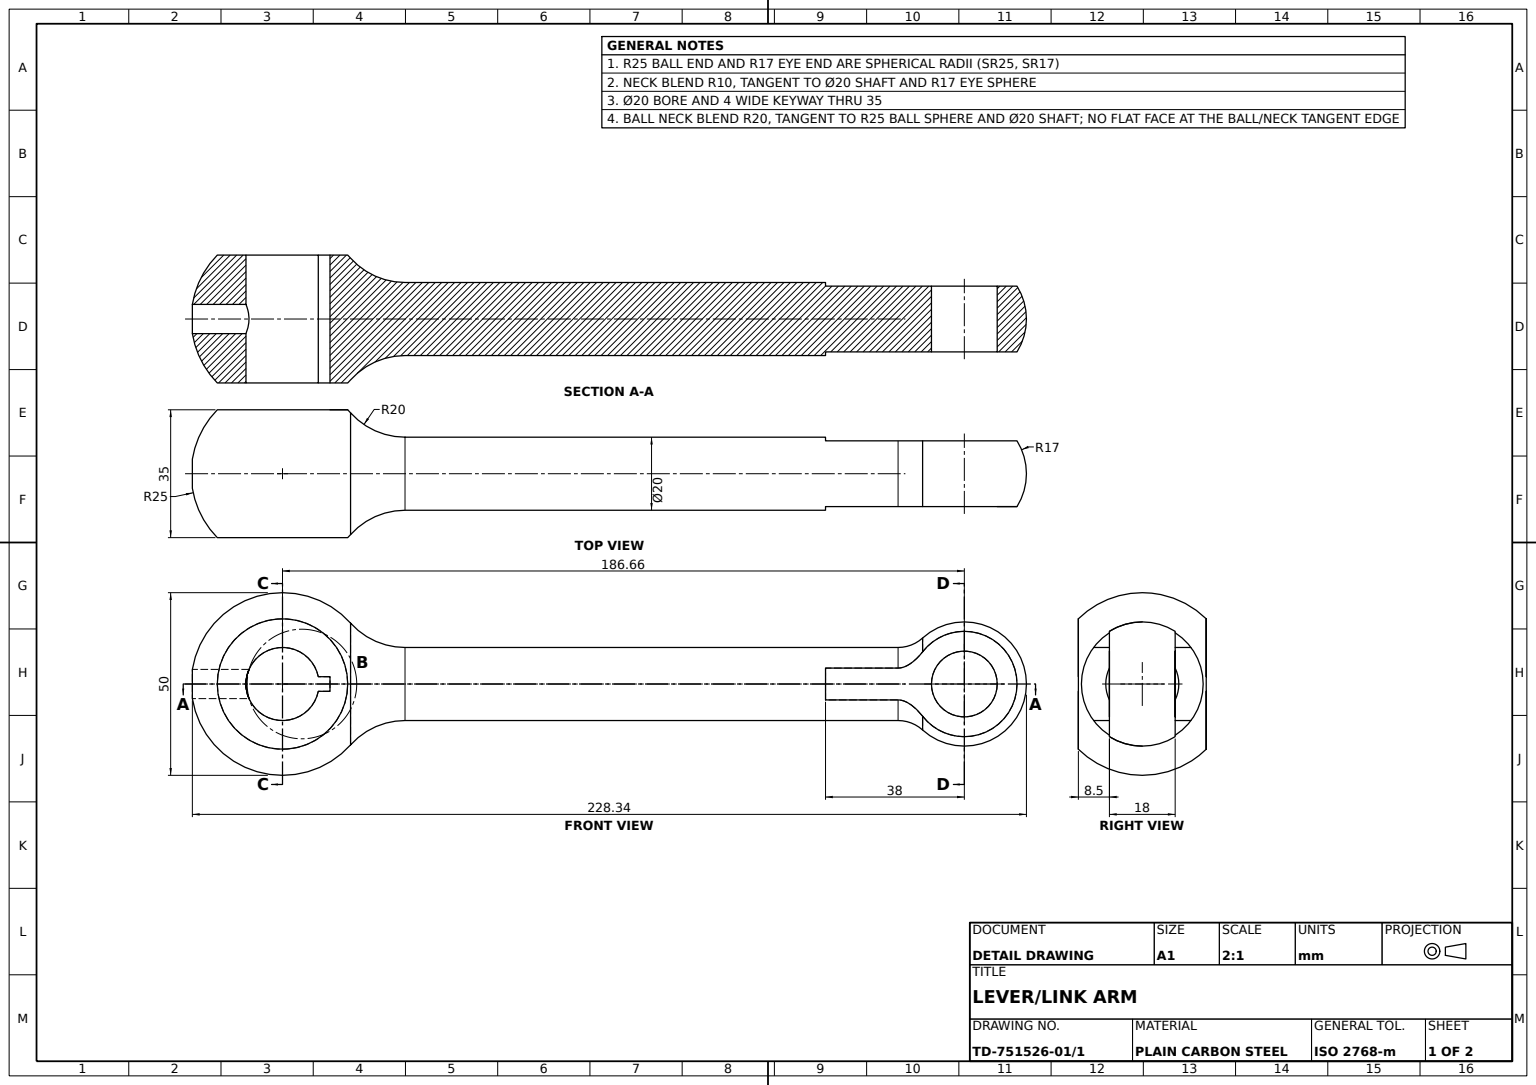
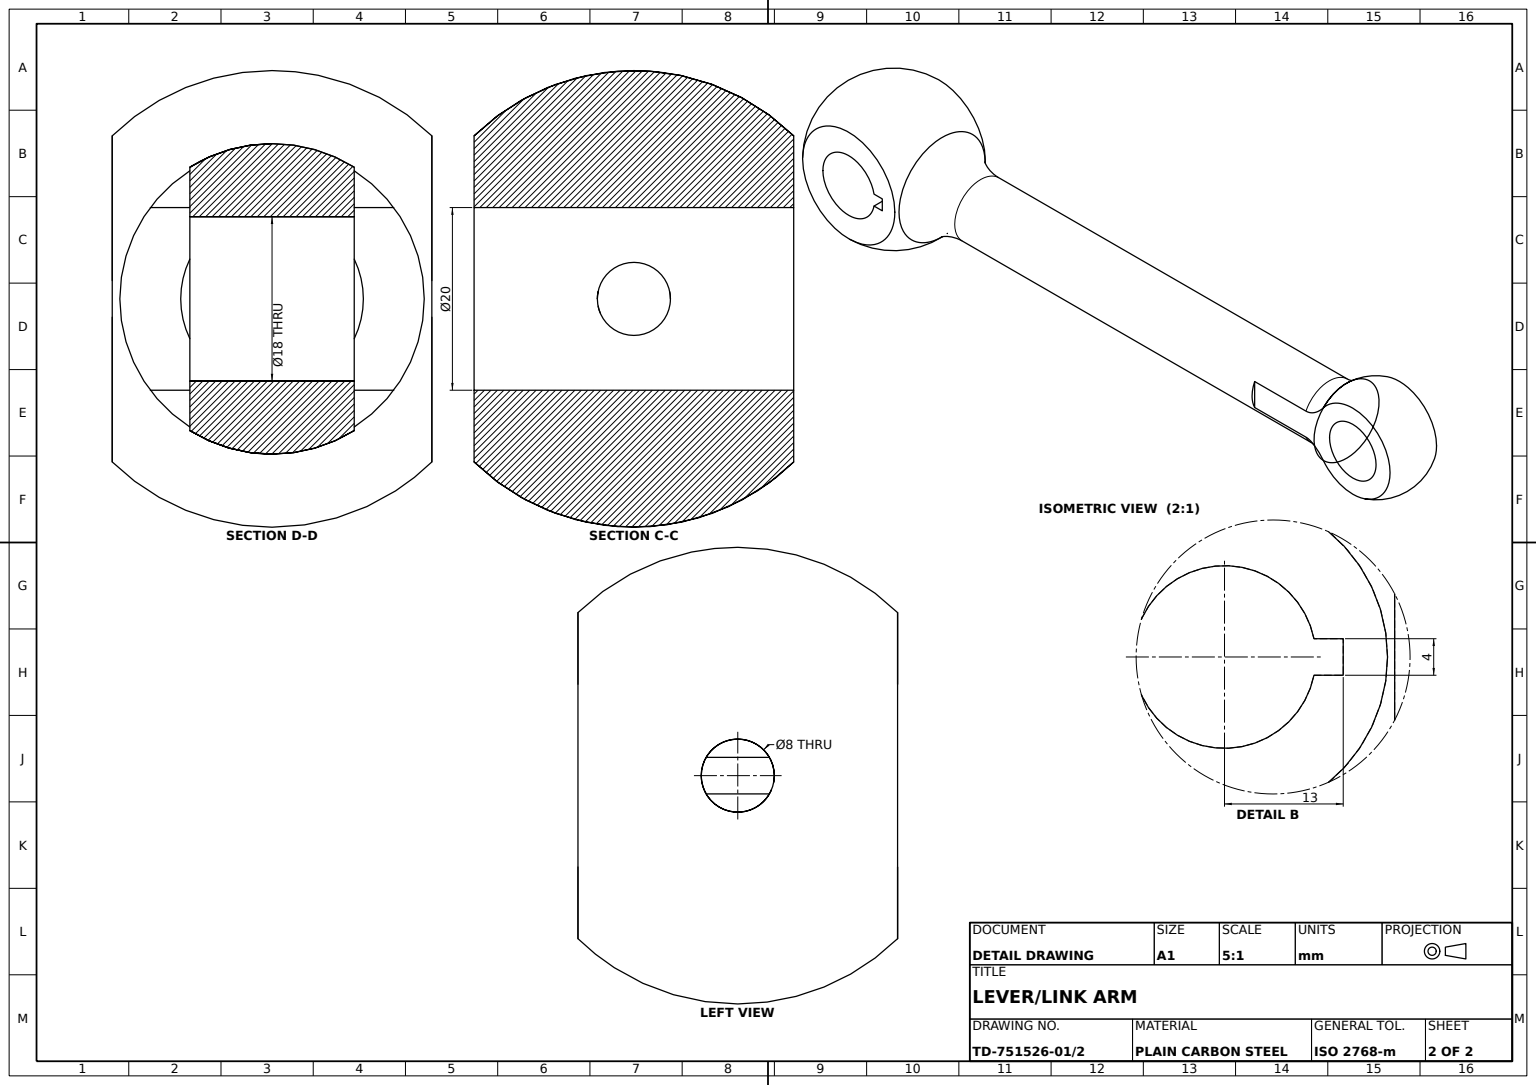
ISO-10303-21;
HEADER;
FILE_DESCRIPTION((''),'2;1');
FILE_NAME('','',(''),(''),'','','');
FILE_SCHEMA(('AUTOMOTIVE_DESIGN'));
ENDSEC;
DATA;
#1=APPLICATION_CONTEXT('');
#2=PRODUCT_CONTEXT('',#1,'mechanical');
#3=PRODUCT('','','',(#2));
#4=PRODUCT_DEFINITION_FORMATION('','',#3);
#5=PRODUCT_DEFINITION_CONTEXT('',#1,'design');
#6=PRODUCT_DEFINITION('','',#4,#5);
#7=PRODUCT_DEFINITION_SHAPE('','',#6);
#8=(LENGTH_UNIT()NAMED_UNIT(*)SI_UNIT(.MILLI.,.METRE.));
#9=(NAMED_UNIT(*)PLANE_ANGLE_UNIT()SI_UNIT($,.RADIAN.));
#10=(NAMED_UNIT(*)SI_UNIT($,.STERADIAN.)SOLID_ANGLE_UNIT());
#11=UNCERTAINTY_MEASURE_WITH_UNIT(LENGTH_MEASURE(1.E-05),#8,'distance_accuracy_value','');
#12=(GEOMETRIC_REPRESENTATION_CONTEXT(3)GLOBAL_UNCERTAINTY_ASSIGNED_CONTEXT((#11))GLOBAL_UNIT_ASSIGNED_CONTEXT((#8,#9,#10))REPRESENTATION_CONTEXT('',''));
#13=CARTESIAN_POINT('',(177.660606,0.,-9.));
#14=VERTEX_POINT('',#13);
#15=CARTESIAN_POINT('',(195.660606,0.,-9.));
#16=VERTEX_POINT('',#15);
#17=CARTESIAN_POINT('',(186.660606,0.,-9.));
#18=DIRECTION('',(0.,0.,-1.));
#19=DIRECTION('',(1.,0.,0.));
#20=AXIS2_PLACEMENT_3D('',#17,#18,#19);
#21=CIRCLE('',#20,9.);
#22=EDGE_CURVE('',#14,#16,#21,.T.);
#23=ORIENTED_EDGE('',*,*,#22,.T.);
#24=CARTESIAN_POINT('',(195.660606,0.,9.));
#25=VERTEX_POINT('',#24);
#26=CARTESIAN_POINT('',(195.660606,0.,-17.501));
#27=DIRECTION('',(0.,0.,1.));
#28=VECTOR('',#27,1000.);
#29=LINE('',#26,#28);
#30=EDGE_CURVE('',#16,#25,#29,.T.);
#31=ORIENTED_EDGE('',*,*,#30,.T.);
#32=CARTESIAN_POINT('',(177.660606,0.,9.));
#33=VERTEX_POINT('',#32);
#34=CARTESIAN_POINT('',(186.660606,0.,9.));
#35=AXIS2_PLACEMENT_3D('',#34,#27,#19);
#36=CIRCLE('',#35,9.);
#37=EDGE_CURVE('',#25,#33,#36,.T.);
#38=ORIENTED_EDGE('',*,*,#37,.T.);
#39=CARTESIAN_POINT('',(177.660606,0.,-17.501));
#40=LINE('',#39,#28);
#41=EDGE_CURVE('',#14,#33,#40,.T.);
#42=ORIENTED_EDGE('',*,*,#41,.F.);
#43=EDGE_LOOP('',(#23,#31,#38,#42));
#44=FACE_OUTER_BOUND('',#43,.T.);
#45=CARTESIAN_POINT('',(186.660606,0.,-17.501));
#46=AXIS2_PLACEMENT_3D('',#45,#27,#19);
#47=CYLINDRICAL_SURFACE('',#46,9.);
#48=ADVANCED_FACE('',(#44),#47,.F.);
#49=CARTESIAN_POINT('',(33.54102,0.,-10.));
#50=VERTEX_POINT('',#49);
#51=CARTESIAN_POINT('',(18.6339,0.,-16.666667));
#52=VERTEX_POINT('',#51);
#53=CARTESIAN_POINT('',(33.54102,0.,-30.));
#54=DIRECTION('',(0.,-1.,0.));
#55=AXIS2_PLACEMENT_3D('',#53,#54,#18);
#56=CIRCLE('',#55,20.);
#57=EDGE_CURVE('',#50,#52,#56,.T.);
#58=ORIENTED_EDGE('',*,*,#57,.T.);
#59=CARTESIAN_POINT('',(18.6339,0.,16.666667));
#60=VERTEX_POINT('',#59);
#61=CARTESIAN_POINT('',(18.6339,0.,0.));
#62=AXIS2_PLACEMENT_3D('',#61,#19,#18);
#63=CIRCLE('',#62,16.666667);
#64=EDGE_CURVE('',#52,#60,#63,.T.);
#65=ORIENTED_EDGE('',*,*,#64,.T.);
#66=CARTESIAN_POINT('',(33.54102,0.,10.));
#67=VERTEX_POINT('',#66);
#68=CARTESIAN_POINT('',(33.54102,0.,30.));
#69=DIRECTION('',(0.,1.,0.));
#70=AXIS2_PLACEMENT_3D('',#68,#69,#27);
#71=CIRCLE('',#70,20.);
#72=EDGE_CURVE('',#67,#60,#71,.T.);
#73=ORIENTED_EDGE('',*,*,#72,.F.);
#74=CARTESIAN_POINT('',(33.54102,0.,0.));
#75=AXIS2_PLACEMENT_3D('',#74,#19,#18);
#76=CIRCLE('',#75,10.);
#77=EDGE_CURVE('',#50,#67,#76,.T.);
#78=ORIENTED_EDGE('',*,*,#77,.F.);
#79=EDGE_LOOP('',(#58,#65,#73,#78));
#80=FACE_OUTER_BOUND('',#79,.T.);
#81=TOROIDAL_SURFACE('',#75,30.,20.);
#82=ADVANCED_FACE('',(#80),#81,.F.);
#83=ORIENTED_EDGE('',*,*,#30,.F.);
#84=EDGE_CURVE('',#16,#14,#21,.T.);
#85=ORIENTED_EDGE('',*,*,#84,.T.);
#86=ORIENTED_EDGE('',*,*,#41,.T.);
#87=EDGE_CURVE('',#33,#25,#36,.T.);
#88=ORIENTED_EDGE('',*,*,#87,.T.);
#89=EDGE_LOOP('',(#83,#85,#86,#88));
#90=FACE_OUTER_BOUND('',#89,.T.);
#91=ADVANCED_FACE('',(#90),#47,.F.);
#92=CARTESIAN_POINT('',(13.,2.,17.5));
#93=VERTEX_POINT('',#92);
#94=CARTESIAN_POINT('',(13.,-2.,17.5));
#95=VERTEX_POINT('',#94);
#96=VECTOR('',#54,1000.);
#97=LINE('',#92,#96);
#98=EDGE_CURVE('',#93,#95,#97,.T.);
#99=ORIENTED_EDGE('',*,*,#98,.F.);
#100=CARTESIAN_POINT('',(13.,2.,-17.5));
#101=VERTEX_POINT('',#100);
#102=CARTESIAN_POINT('',(13.,2.,17.501));
#103=VECTOR('',#18,1000.);
#104=LINE('',#102,#103);
#105=EDGE_CURVE('',#93,#101,#104,.T.);
#106=ORIENTED_EDGE('',*,*,#105,.T.);
#107=CARTESIAN_POINT('',(13.,-2.,-17.5));
#108=VERTEX_POINT('',#107);
#109=LINE('',#100,#96);
#110=EDGE_CURVE('',#101,#108,#109,.T.);
#111=ORIENTED_EDGE('',*,*,#110,.T.);
#112=CARTESIAN_POINT('',(13.,-2.,17.501));
#113=LINE('',#112,#103);
#114=EDGE_CURVE('',#95,#108,#113,.T.);
#115=ORIENTED_EDGE('',*,*,#114,.F.);
#116=EDGE_LOOP('',(#99,#106,#111,#115));
#117=FACE_OUTER_BOUND('',#116,.T.);
#118=AXIS2_PLACEMENT_3D('',#102,#19,#18);
#119=PLANE('',#118);
#120=ADVANCED_FACE('',(#117),#119,.F.);
#121=CARTESIAN_POINT('',(168.522248,4.358899,-9.));
#122=VERTEX_POINT('',#121);
#123=CARTESIAN_POINT('',(168.522248,4.358899,9.));
#124=VERTEX_POINT('',#123);
#125=CARTESIAN_POINT('',(168.522248,0.,0.));
#126=AXIS2_PLACEMENT_3D('',#125,#19,#18);
#127=CIRCLE('',#126,10.);
#128=EDGE_CURVE('',#122,#124,#127,.T.);
#129=ORIENTED_EDGE('',*,*,#128,.T.);
#130=CARTESIAN_POINT('',(175.240158,8.807576,9.));
#131=VERTEX_POINT('',#130);
#132=CARTESIAN_POINT('',(168.874076,4.358899,9.));
#133=CARTESIAN_POINT('',(169.21845,4.401685,9.));
#134=CARTESIAN_POINT('',(169.894624,4.559455,9.));
#135=CARTESIAN_POINT('',(170.22884,4.675527,9.));
#136=CARTESIAN_POINT('',(170.870066,4.956873,9.));
#137=CARTESIAN_POINT('',(171.175147,5.120207,9.));
#138=CARTESIAN_POINT('',(171.763901,5.478102,9.));
#139=CARTESIAN_POINT('',(172.047475,5.672809,9.));
#140=CARTESIAN_POINT('',(172.598036,6.086423,9.));
#141=CARTESIAN_POINT('',(172.864975,6.305399,9.));
#142=CARTESIAN_POINT('',(173.384701,6.763997,9.));
#143=CARTESIAN_POINT('',(173.638132,7.004413,9.));
#144=CARTESIAN_POINT('',(174.369091,7.744052,9.));
#145=CARTESIAN_POINT('',(174.820762,8.26376,9.));
#146=B_SPLINE_CURVE_WITH_KNOTS('',3,(#123,#132,#133,#134,#135,#136,#137,#138,#139,#140,#141,#142,#143,#144,#145,#130),.UNSPECIFIED.,.F.,.F.,(4,2,2,2,2,2,2,4),(0.066540398,0.067572352,0.068604305,0.069636258,0.070668212,0.071700165,0.072732118,0.074796025),.UNSPECIFIED.);
#147=EDGE_CURVE('',#124,#131,#146,.T.);
#148=ORIENTED_EDGE('',*,*,#147,.T.);
#149=CARTESIAN_POINT('',(175.240158,8.807576,-9.));
#150=VERTEX_POINT('',#149);
#151=CARTESIAN_POINT('',(175.240158,0.,0.));
#152=AXIS2_PLACEMENT_3D('',#151,#19,#18);
#153=CIRCLE('',#152,12.592593);
#154=EDGE_CURVE('',#150,#131,#153,.T.);
#155=ORIENTED_EDGE('',*,*,#154,.F.);
#156=CARTESIAN_POINT('',(168.874076,4.358899,-9.));
#157=CARTESIAN_POINT('',(169.21845,4.401685,-9.));
#158=CARTESIAN_POINT('',(169.894624,4.559455,-9.));
#159=CARTESIAN_POINT('',(170.22884,4.675527,-9.));
#160=CARTESIAN_POINT('',(170.870066,4.956873,-9.));
#161=CARTESIAN_POINT('',(171.175147,5.120207,-9.));
#162=CARTESIAN_POINT('',(171.763901,5.478102,-9.));
#163=CARTESIAN_POINT('',(172.047475,5.672809,-9.));
#164=CARTESIAN_POINT('',(172.598036,6.086423,-9.));
#165=CARTESIAN_POINT('',(172.864975,6.305399,-9.));
#166=CARTESIAN_POINT('',(173.384701,6.763997,-9.));
#167=CARTESIAN_POINT('',(173.638132,7.004413,-9.));
#168=CARTESIAN_POINT('',(174.369091,7.744052,-9.));
#169=CARTESIAN_POINT('',(174.820762,8.26376,-9.));
#170=B_SPLINE_CURVE_WITH_KNOTS('',3,(#121,#156,#157,#158,#159,#160,#161,#162,#163,#164,#165,#166,#167,#168,#169,#149),.UNSPECIFIED.,.F.,.F.,(4,2,2,2,2,2,2,4),(0.066540398,0.067572352,0.068604305,0.069636258,0.070668212,0.071700165,0.072732118,0.074796025),.UNSPECIFIED.);
#171=EDGE_CURVE('',#122,#150,#170,.T.);
#172=ORIENTED_EDGE('',*,*,#171,.F.);
#173=EDGE_LOOP('',(#129,#148,#155,#172));
#174=FACE_OUTER_BOUND('',#173,.T.);
#175=TOROIDAL_SURFACE('',#126,20.,10.);
#176=ADVANCED_FACE('',(#174),#175,.F.);
#177=CARTESIAN_POINT('',(-24.677925,0.,-4.));
#178=VERTEX_POINT('',#177);
#179=CARTESIAN_POINT('',(-17.853571,0.,-17.5));
#180=VERTEX_POINT('',#179);
#181=CARTESIAN_POINT('',(0.,0.,0.));
#182=AXIS2_PLACEMENT_3D('',#181,#54,#18);
#183=CIRCLE('',#182,25.);
#184=EDGE_CURVE('',#178,#180,#183,.T.);
#185=ORIENTED_EDGE('',*,*,#184,.F.);
#186=CARTESIAN_POINT('',(-24.677925,0.,4.));
#187=VERTEX_POINT('',#186);
#188=CARTESIAN_POINT('',(-24.677925,0.,0.));
#189=DIRECTION('',(-1.,0.,0.));
#190=AXIS2_PLACEMENT_3D('',#188,#189,#18);
#191=CIRCLE('',#190,4.);
#192=EDGE_CURVE('',#187,#178,#191,.T.);
#193=ORIENTED_EDGE('',*,*,#192,.F.);
#194=CARTESIAN_POINT('',(-17.853571,0.,17.5));
#195=VERTEX_POINT('',#194);
#196=AXIS2_PLACEMENT_3D('',#181,#69,#27);
#197=CIRCLE('',#196,25.);
#198=EDGE_CURVE('',#187,#195,#197,.T.);
#199=ORIENTED_EDGE('',*,*,#198,.T.);
#200=CARTESIAN_POINT('',(17.853571,0.,17.5));
#201=VERTEX_POINT('',#200);
#202=CARTESIAN_POINT('',(0.,0.,17.5));
#203=AXIS2_PLACEMENT_3D('',#202,#27,#19);
#204=CIRCLE('',#203,17.853571);
#205=EDGE_CURVE('',#201,#195,#204,.T.);
#206=ORIENTED_EDGE('',*,*,#205,.F.);
#207=EDGE_CURVE('',#201,#60,#197,.T.);
#208=ORIENTED_EDGE('',*,*,#207,.T.);
#209=ORIENTED_EDGE('',*,*,#64,.F.);
#210=CARTESIAN_POINT('',(17.853571,0.,-17.5));
#211=VERTEX_POINT('',#210);
#212=EDGE_CURVE('',#211,#52,#183,.T.);
#213=ORIENTED_EDGE('',*,*,#212,.F.);
#214=CARTESIAN_POINT('',(0.,0.,-17.5));
#215=AXIS2_PLACEMENT_3D('',#214,#27,#19);
#216=CIRCLE('',#215,17.853571);
#217=EDGE_CURVE('',#211,#180,#216,.T.);
#218=ORIENTED_EDGE('',*,*,#217,.T.);
#219=EDGE_LOOP('',(#185,#193,#199,#206,#208,#209,#213,#218));
#220=FACE_OUTER_BOUND('',#219,.T.);
#221=AXIS2_PLACEMENT_3D('',#181,#69,#18);
#222=SPHERICAL_SURFACE('',#221,25.);
#223=ADVANCED_FACE('',(#220),#222,.T.);
#224=ORIENTED_EDGE('',*,*,#22,.F.);
#225=ORIENTED_EDGE('',*,*,#84,.F.);
#226=EDGE_LOOP('',(#224,#225));
#227=FACE_BOUND('',#226,.T.);
#228=CARTESIAN_POINT('',(148.660606,4.358899,-9.));
#229=VERTEX_POINT('',#228);
#230=CARTESIAN_POINT('',(248.139692,4.358899,-9.));
#231=VECTOR('',#19,1000.);
#232=LINE('',#230,#231);
#233=EDGE_CURVE('',#229,#122,#232,.T.);
#234=ORIENTED_EDGE('',*,*,#233,.T.);
#235=ORIENTED_EDGE('',*,*,#171,.T.);
#236=CARTESIAN_POINT('',(201.082811,0.,-9.));
#237=VERTEX_POINT('',#236);
#238=CIRCLE('',#20,14.422205);
#239=EDGE_CURVE('',#150,#237,#238,.T.);
#240=ORIENTED_EDGE('',*,*,#239,.T.);
#241=CARTESIAN_POINT('',(175.240158,-8.807576,-9.));
#242=VERTEX_POINT('',#241);
#243=EDGE_CURVE('',#237,#242,#238,.T.);
#244=ORIENTED_EDGE('',*,*,#243,.T.);
#245=CARTESIAN_POINT('',(168.522248,-4.358899,-9.));
#246=VERTEX_POINT('',#245);
#247=CARTESIAN_POINT('',(174.81656,-8.258312,-9.));
#248=CARTESIAN_POINT('',(174.36214,-7.736405,-9.));
#249=CARTESIAN_POINT('',(173.38727,-6.751194,-9.));
#250=CARTESIAN_POINT('',(172.867869,-6.288445,-9.));
#251=CARTESIAN_POINT('',(172.038646,-5.66653,-9.));
#252=CARTESIAN_POINT('',(171.753259,-5.470946,-9.));
#253=CARTESIAN_POINT('',(171.158648,-5.110896,-9.));
#254=CARTESIAN_POINT('',(170.85143,-4.94783,-9.));
#255=CARTESIAN_POINT('',(170.218697,-4.671983,-9.));
#256=CARTESIAN_POINT('',(169.892126,-4.558498,-9.));
#257=CARTESIAN_POINT('',(169.210806,-4.400281,-9.));
#258=CARTESIAN_POINT('',(168.867809,-4.358899,-9.));
#259=B_SPLINE_CURVE_WITH_KNOTS('',3,(#241,#247,#248,#249,#250,#251,#252,#253,#254,#255,#256,#257,#258,#245),.UNSPECIFIED.,.F.,.F.,(4,2,2,2,2,2,4),(0.066419466,0.068492414,0.070565363,0.071601837,0.072638311,0.073674786,0.07471126),.UNSPECIFIED.);
#260=EDGE_CURVE('',#242,#246,#259,.T.);
#261=ORIENTED_EDGE('',*,*,#260,.T.);
#262=CARTESIAN_POINT('',(148.660606,-4.358899,-9.));
#263=VERTEX_POINT('',#262);
#264=CARTESIAN_POINT('',(248.139692,-4.358899,-9.));
#265=VECTOR('',#189,1000.);
#266=LINE('',#264,#265);
#267=EDGE_CURVE('',#246,#263,#266,.T.);
#268=ORIENTED_EDGE('',*,*,#267,.T.);
#269=CARTESIAN_POINT('',(148.660606,5.,-9.));
#270=LINE('',#269,#96);
#271=EDGE_CURVE('',#229,#263,#270,.T.);
#272=ORIENTED_EDGE('',*,*,#271,.F.);
#273=EDGE_LOOP('',(#234,#235,#240,#244,#261,#268,#272));
#274=FACE_OUTER_BOUND('',#273,.T.);
#275=AXIS2_PLACEMENT_3D('',#17,#27,#19);
#276=PLANE('',#275);
#277=ADVANCED_FACE('',(#227,#274),#276,.F.);
#278=CARTESIAN_POINT('',(9.797959,-2.,17.5));
#279=VERTEX_POINT('',#278);
#280=LINE('',#94,#265);
#281=EDGE_CURVE('',#95,#279,#280,.T.);
#282=ORIENTED_EDGE('',*,*,#281,.F.);
#283=ORIENTED_EDGE('',*,*,#114,.T.);
#284=CARTESIAN_POINT('',(9.797959,-2.,-17.5));
#285=VERTEX_POINT('',#284);
#286=LINE('',#107,#265);
#287=EDGE_CURVE('',#108,#285,#286,.T.);
#288=ORIENTED_EDGE('',*,*,#287,.T.);
#289=CARTESIAN_POINT('',(9.797959,-2.,17.501));
#290=LINE('',#289,#103);
#291=EDGE_CURVE('',#279,#285,#290,.T.);
#292=ORIENTED_EDGE('',*,*,#291,.F.);
#293=EDGE_LOOP('',(#282,#283,#288,#292));
#294=FACE_OUTER_BOUND('',#293,.T.);
#295=AXIS2_PLACEMENT_3D('',#112,#54,#18);
#296=PLANE('',#295);
#297=ADVANCED_FACE('',(#294),#296,.F.);
#298=CARTESIAN_POINT('',(168.522248,-4.358899,9.));
#299=VERTEX_POINT('',#298);
#300=CARTESIAN_POINT('',(148.660606,-4.358899,9.));
#301=VERTEX_POINT('',#300);
#302=CARTESIAN_POINT('',(248.139692,-4.358899,9.));
#303=LINE('',#302,#265);
#304=EDGE_CURVE('',#299,#301,#303,.T.);
#305=ORIENTED_EDGE('',*,*,#304,.F.);
#306=CARTESIAN_POINT('',(175.240158,-8.807576,9.));
#307=VERTEX_POINT('',#306);
#308=CARTESIAN_POINT('',(174.81656,-8.258312,9.));
#309=CARTESIAN_POINT('',(174.36214,-7.736405,9.));
#310=CARTESIAN_POINT('',(173.38727,-6.751194,9.));
#311=CARTESIAN_POINT('',(172.867869,-6.288445,9.));
#312=CARTESIAN_POINT('',(172.038646,-5.66653,9.));
#313=CARTESIAN_POINT('',(171.753259,-5.470946,9.));
#314=CARTESIAN_POINT('',(171.158648,-5.110896,9.));
#315=CARTESIAN_POINT('',(170.85143,-4.94783,9.));
#316=CARTESIAN_POINT('',(170.218697,-4.671983,9.));
#317=CARTESIAN_POINT('',(169.892126,-4.558498,9.));
#318=CARTESIAN_POINT('',(169.210806,-4.400281,9.));
#319=CARTESIAN_POINT('',(168.867809,-4.358899,9.));
#320=B_SPLINE_CURVE_WITH_KNOTS('',3,(#306,#308,#309,#310,#311,#312,#313,#314,#315,#316,#317,#318,#319,#298),.UNSPECIFIED.,.F.,.F.,(4,2,2,2,2,2,4),(0.066419466,0.068492414,0.070565363,0.071601837,0.072638311,0.073674786,0.07471126),.UNSPECIFIED.);
#321=EDGE_CURVE('',#307,#299,#320,.T.);
#322=ORIENTED_EDGE('',*,*,#321,.F.);
#323=CARTESIAN_POINT('',(201.082811,0.,9.));
#324=VERTEX_POINT('',#323);
#325=AXIS2_PLACEMENT_3D('',#34,#18,#19);
#326=CIRCLE('',#325,14.422205);
#327=EDGE_CURVE('',#324,#307,#326,.T.);
#328=ORIENTED_EDGE('',*,*,#327,.F.);
#329=EDGE_CURVE('',#131,#324,#326,.T.);
#330=ORIENTED_EDGE('',*,*,#329,.F.);
#331=ORIENTED_EDGE('',*,*,#147,.F.);
#332=CARTESIAN_POINT('',(148.660606,4.358899,9.));
#333=VERTEX_POINT('',#332);
#334=CARTESIAN_POINT('',(248.139692,4.358899,9.));
#335=LINE('',#334,#231);
#336=EDGE_CURVE('',#333,#124,#335,.T.);
#337=ORIENTED_EDGE('',*,*,#336,.F.);
#338=CARTESIAN_POINT('',(148.660606,5.,9.));
#339=LINE('',#338,#96);
#340=EDGE_CURVE('',#333,#301,#339,.T.);
#341=ORIENTED_EDGE('',*,*,#340,.T.);
#342=EDGE_LOOP('',(#305,#322,#328,#330,#331,#337,#341));
#343=FACE_OUTER_BOUND('',#342,.T.);
#344=ORIENTED_EDGE('',*,*,#87,.F.);
#345=ORIENTED_EDGE('',*,*,#37,.F.);
#346=EDGE_LOOP('',(#344,#345));
#347=FACE_BOUND('',#346,.T.);
#348=PLANE('',#35);
#349=ADVANCED_FACE('',(#343,#347),#348,.T.);
#350=ORIENTED_EDGE('',*,*,#271,.T.);
#351=CARTESIAN_POINT('',(148.660606,0.,-10.));
#352=VERTEX_POINT('',#351);
#353=CARTESIAN_POINT('',(148.660606,0.,0.));
#354=AXIS2_PLACEMENT_3D('',#353,#19,#27);
#355=CIRCLE('',#354,10.);
#356=EDGE_CURVE('',#263,#352,#355,.T.);
#357=ORIENTED_EDGE('',*,*,#356,.T.);
#358=EDGE_CURVE('',#352,#229,#355,.T.);
#359=ORIENTED_EDGE('',*,*,#358,.T.);
#360=EDGE_LOOP('',(#350,#357,#359));
#361=FACE_OUTER_BOUND('',#360,.T.);
#362=CARTESIAN_POINT('',(148.660606,5.,-17.501));
#363=AXIS2_PLACEMENT_3D('',#362,#189,#27);
#364=PLANE('',#363);
#365=ADVANCED_FACE('',(#361),#364,.F.);
#366=EDGE_CURVE('',#60,#52,#63,.T.);
#367=ORIENTED_EDGE('',*,*,#366,.T.);
#368=ORIENTED_EDGE('',*,*,#57,.F.);
#369=EDGE_CURVE('',#67,#50,#76,.T.);
#370=ORIENTED_EDGE('',*,*,#369,.F.);
#371=ORIENTED_EDGE('',*,*,#72,.T.);
#372=EDGE_LOOP('',(#367,#368,#370,#371));
#373=FACE_OUTER_BOUND('',#372,.T.);
#374=ADVANCED_FACE('',(#373),#81,.F.);
#375=EDGE_CURVE('',#299,#246,#127,.T.);
#376=ORIENTED_EDGE('',*,*,#375,.T.);
#377=ORIENTED_EDGE('',*,*,#260,.F.);
#378=EDGE_CURVE('',#307,#242,#153,.T.);
#379=ORIENTED_EDGE('',*,*,#378,.F.);
#380=ORIENTED_EDGE('',*,*,#321,.T.);
#381=EDGE_LOOP('',(#376,#377,#379,#380));
#382=FACE_OUTER_BOUND('',#381,.T.);
#383=ADVANCED_FACE('',(#382),#175,.F.);
#384=CARTESIAN_POINT('',(-10.,0.,4.));
#385=VERTEX_POINT('',#384);
#386=CARTESIAN_POINT('',(-10.,0.,-4.));
#387=VERTEX_POINT('',#386);
#388=CARTESIAN_POINT('',(-10.,-0.263112,4.));
#389=CARTESIAN_POINT('',(-9.989336,-0.52985,3.973555));
#390=CARTESIAN_POINT('',(-9.948313,-1.048164,3.869268));
#391=CARTESIAN_POINT('',(-9.918356,-1.298524,3.792435));
#392=CARTESIAN_POINT('',(-9.842917,-1.782398,3.590513));
#393=CARTESIAN_POINT('',(-9.797311,-2.015291,3.464932));
#394=CARTESIAN_POINT('',(-9.698876,-2.445507,3.175948));
#395=CARTESIAN_POINT('',(-9.645461,-2.646134,3.010987));
#396=CARTESIAN_POINT('',(-9.536652,-3.014832,2.641753));
#397=CARTESIAN_POINT('',(-9.482634,-3.178513,2.442105));
#398=CARTESIAN_POINT('',(-9.381221,-3.466408,2.012671));
#399=CARTESIAN_POINT('',(-9.333353,-3.591691,1.779932));
#400=CARTESIAN_POINT('',(-9.25342,-3.792879,1.2971));
#401=CARTESIAN_POINT('',(-9.221268,-3.86929,1.047714));
#402=CARTESIAN_POINT('',(-9.177005,-3.973131,0.532297));
#403=CARTESIAN_POINT('',(-9.165166,-3.999967,0.264113));
#404=CARTESIAN_POINT('',(-9.165137,-4.000033,-0.263104));
#405=CARTESIAN_POINT('',(-9.176515,-3.974265,-0.525135));
#406=CARTESIAN_POINT('',(-9.220997,-3.869938,-1.046004));
#407=CARTESIAN_POINT('',(-9.253578,-3.792487,-1.298117));
#408=CARTESIAN_POINT('',(-9.33333,-3.591742,-1.779734));
#409=CARTESIAN_POINT('',(-9.381197,-3.46651,-2.012662));
#410=CARTESIAN_POINT('',(-9.483143,-3.177034,-2.444167));
#411=CARTESIAN_POINT('',(-9.537174,-3.013117,-2.643571));
#412=CARTESIAN_POINT('',(-9.645399,-2.646291,-3.010729));
#413=CARTESIAN_POINT('',(-9.699402,-2.443392,-3.177539));
#414=CARTESIAN_POINT('',(-9.797619,-2.013759,-3.465789));
#415=CARTESIAN_POINT('',(-9.842453,-1.785184,-3.58926));
#416=CARTESIAN_POINT('',(-9.918457,-1.298068,-3.792715));
#417=CARTESIAN_POINT('',(-9.948453,-1.046303,-3.869623));
#418=CARTESIAN_POINT('',(-9.989151,-0.532292,-3.973084));
#419=CARTESIAN_POINT('',(-10.,-0.267133,-4.));
#420=B_SPLINE_CURVE_WITH_KNOTS('',3,(#384,#388,#389,#390,#391,#392,#393,#394,#395,#396,#397,#398,#399,#400,#401,#402,#403,#404,#405,#406,#407,#408,#409,#410,#411,#412,#413,#414,#415,#416,#417,#418,#419,#386),.UNSPECIFIED.,.F.,.F.,(4,2,2,2,2,2,2,2,2,2,2,2,2,2,2,2,4),(0.012639562,0.013429016,0.014218471,0.015007925,0.015797379,0.016586833,0.017376287,0.018165741,0.018955196,0.01974465,0.020534104,0.021323558,0.022113012,0.022902467,0.023691921,0.024481375,0.025270829),.UNSPECIFIED.);
#421=EDGE_CURVE('',#385,#387,#420,.T.);
#422=ORIENTED_EDGE('',*,*,#421,.F.);
#423=CARTESIAN_POINT('',(-10.,0.,17.5));
#424=VERTEX_POINT('',#423);
#425=CARTESIAN_POINT('',(-10.,0.,17.501));
#426=LINE('',#425,#103);
#427=EDGE_CURVE('',#424,#385,#426,.T.);
#428=ORIENTED_EDGE('',*,*,#427,.F.);
#429=AXIS2_PLACEMENT_3D('',#202,#18,#19);
#430=CIRCLE('',#429,10.);
#431=EDGE_CURVE('',#279,#424,#430,.T.);
#432=ORIENTED_EDGE('',*,*,#431,.F.);
#433=ORIENTED_EDGE('',*,*,#291,.T.);
#434=CARTESIAN_POINT('',(-10.,0.,-17.5));
#435=VERTEX_POINT('',#434);
#436=AXIS2_PLACEMENT_3D('',#214,#18,#189);
#437=CIRCLE('',#436,10.);
#438=EDGE_CURVE('',#285,#435,#437,.T.);
#439=ORIENTED_EDGE('',*,*,#438,.T.);
#440=EDGE_CURVE('',#387,#435,#426,.T.);
#441=ORIENTED_EDGE('',*,*,#440,.F.);
#442=EDGE_LOOP('',(#422,#428,#432,#433,#439,#441));
#443=FACE_OUTER_BOUND('',#442,.T.);
#444=CARTESIAN_POINT('',(0.,0.,17.501));
#445=AXIS2_PLACEMENT_3D('',#444,#18,#189);
#446=CYLINDRICAL_SURFACE('',#445,10.);
#447=ADVANCED_FACE('',(#443),#446,.F.);
#448=ORIENTED_EDGE('',*,*,#243,.F.);
#449=CARTESIAN_POINT('',(203.660606,0.,0.));
#450=VERTEX_POINT('',#449);
#451=CARTESIAN_POINT('',(186.660606,0.,0.));
#452=AXIS2_PLACEMENT_3D('',#451,#54,#18);
#453=CIRCLE('',#452,17.);
#454=EDGE_CURVE('',#237,#450,#453,.T.);
#455=ORIENTED_EDGE('',*,*,#454,.T.);
#456=AXIS2_PLACEMENT_3D('',#451,#69,#27);
#457=CIRCLE('',#456,17.);
#458=EDGE_CURVE('',#324,#450,#457,.T.);
#459=ORIENTED_EDGE('',*,*,#458,.F.);
#460=ORIENTED_EDGE('',*,*,#327,.T.);
#461=ORIENTED_EDGE('',*,*,#378,.T.);
#462=EDGE_LOOP('',(#448,#455,#459,#460,#461));
#463=FACE_OUTER_BOUND('',#462,.T.);
#464=AXIS2_PLACEMENT_3D('',#451,#54,#27);
#465=SPHERICAL_SURFACE('',#464,17.);
#466=ADVANCED_FACE('',(#463),#465,.T.);
#467=CARTESIAN_POINT('',(148.660606,0.,10.));
#468=VERTEX_POINT('',#467);
#469=AXIS2_PLACEMENT_3D('',#353,#189,#18);
#470=CIRCLE('',#469,10.);
#471=EDGE_CURVE('',#301,#468,#470,.T.);
#472=ORIENTED_EDGE('',*,*,#471,.T.);
#473=CARTESIAN_POINT('',(248.139692,0.,10.));
#474=LINE('',#473,#231);
#475=EDGE_CURVE('',#67,#468,#474,.T.);
#476=ORIENTED_EDGE('',*,*,#475,.F.);
#477=ORIENTED_EDGE('',*,*,#369,.T.);
#478=CARTESIAN_POINT('',(248.139692,0.,-10.));
#479=LINE('',#478,#231);
#480=EDGE_CURVE('',#50,#352,#479,.T.);
#481=ORIENTED_EDGE('',*,*,#480,.T.);
#482=ORIENTED_EDGE('',*,*,#356,.F.);
#483=ORIENTED_EDGE('',*,*,#267,.F.);
#484=ORIENTED_EDGE('',*,*,#375,.F.);
#485=ORIENTED_EDGE('',*,*,#304,.T.);
#486=EDGE_LOOP('',(#472,#476,#477,#481,#482,#483,#484,#485));
#487=FACE_OUTER_BOUND('',#486,.T.);
#488=CARTESIAN_POINT('',(248.139692,0.,0.));
#489=AXIS2_PLACEMENT_3D('',#488,#19,#18);
#490=CYLINDRICAL_SURFACE('',#489,10.);
#491=ADVANCED_FACE('',(#487),#490,.T.);
#492=ORIENTED_EDGE('',*,*,#154,.T.);
#493=ORIENTED_EDGE('',*,*,#329,.T.);
#494=ORIENTED_EDGE('',*,*,#458,.T.);
#495=ORIENTED_EDGE('',*,*,#454,.F.);
#496=ORIENTED_EDGE('',*,*,#239,.F.);
#497=EDGE_LOOP('',(#492,#493,#494,#495,#496));
#498=FACE_OUTER_BOUND('',#497,.T.);
#499=ADVANCED_FACE('',(#498),#465,.T.);
#500=ORIENTED_EDGE('',*,*,#217,.F.);
#501=EDGE_CURVE('',#180,#211,#216,.T.);
#502=ORIENTED_EDGE('',*,*,#501,.F.);
#503=EDGE_LOOP('',(#500,#502));
#504=FACE_OUTER_BOUND('',#503,.T.);
#505=CARTESIAN_POINT('',(9.797959,2.,-17.5));
#506=VERTEX_POINT('',#505);
#507=LINE('',#100,#231);
#508=EDGE_CURVE('',#506,#101,#507,.T.);
#509=ORIENTED_EDGE('',*,*,#508,.F.);
#510=EDGE_CURVE('',#435,#506,#437,.T.);
#511=ORIENTED_EDGE('',*,*,#510,.F.);
#512=ORIENTED_EDGE('',*,*,#438,.F.);
#513=ORIENTED_EDGE('',*,*,#287,.F.);
#514=ORIENTED_EDGE('',*,*,#110,.F.);
#515=EDGE_LOOP('',(#509,#511,#512,#513,#514));
#516=FACE_BOUND('',#515,.T.);
#517=PLANE('',#215);
#518=ADVANCED_FACE('',(#504,#516),#517,.F.);
#519=ORIENTED_EDGE('',*,*,#508,.T.);
#520=ORIENTED_EDGE('',*,*,#105,.F.);
#521=CARTESIAN_POINT('',(9.797959,2.,17.5));
#522=VERTEX_POINT('',#521);
#523=LINE('',#92,#231);
#524=EDGE_CURVE('',#522,#93,#523,.T.);
#525=ORIENTED_EDGE('',*,*,#524,.F.);
#526=CARTESIAN_POINT('',(9.797959,2.,17.501));
#527=LINE('',#526,#103);
#528=EDGE_CURVE('',#522,#506,#527,.T.);
#529=ORIENTED_EDGE('',*,*,#528,.T.);
#530=EDGE_LOOP('',(#519,#520,#525,#529));
#531=FACE_OUTER_BOUND('',#530,.T.);
#532=AXIS2_PLACEMENT_3D('',#102,#69,#27);
#533=PLANE('',#532);
#534=ADVANCED_FACE('',(#531),#533,.F.);
#535=CARTESIAN_POINT('',(-10.,0.267309,-4.));
#536=CARTESIAN_POINT('',(-9.989308,0.529624,-3.973479));
#537=CARTESIAN_POINT('',(-9.948623,1.044835,-3.870059));
#538=CARTESIAN_POINT('',(-9.918099,1.300446,-3.791762));
#539=CARTESIAN_POINT('',(-9.842648,1.783852,-3.589776));
#540=CARTESIAN_POINT('',(-9.797885,2.012642,-3.466582));
#541=CARTESIAN_POINT('',(-9.698923,2.445438,-3.176122));
#542=CARTESIAN_POINT('',(-9.644943,2.647871,-3.009215));
#543=CARTESIAN_POINT('',(-9.53732,3.012587,-2.644033));
#544=CARTESIAN_POINT('',(-9.482984,3.177553,-2.443683));
#545=CARTESIAN_POINT('',(-9.380383,3.468752,-2.009027));
#546=CARTESIAN_POINT('',(-9.333486,3.591329,-1.780449));
#547=CARTESIAN_POINT('',(-9.253918,3.791651,-1.300396));
#548=CARTESIAN_POINT('',(-9.220996,3.869938,-1.045589));
#549=CARTESIAN_POINT('',(-9.176724,3.973779,-0.527973));
#550=CARTESIAN_POINT('',(-9.165222,3.999838,-0.266536));
#551=CARTESIAN_POINT('',(-9.165081,4.00016,0.261661));
#552=CARTESIAN_POINT('',(-9.176855,3.973474,0.529767));
#553=CARTESIAN_POINT('',(-9.221002,3.86992,1.045403));
#554=CARTESIAN_POINT('',(-9.253285,3.793242,1.296536));
#555=CARTESIAN_POINT('',(-9.334035,3.589953,1.783796));
#556=CARTESIAN_POINT('',(-9.381199,3.466486,2.012624));
#557=CARTESIAN_POINT('',(-9.482895,3.177756,2.443163));
#558=CARTESIAN_POINT('',(-9.537994,3.0105,2.646488));
#559=CARTESIAN_POINT('',(-9.645941,2.644289,3.012431));
#560=CARTESIAN_POINT('',(-9.699023,2.445017,3.17642));
#561=CARTESIAN_POINT('',(-9.797858,2.012744,3.466499));
#562=CARTESIAN_POINT('',(-9.843385,1.779603,3.591778));
#563=CARTESIAN_POINT('',(-9.918293,1.298724,3.792252));
#564=CARTESIAN_POINT('',(-9.948307,1.048592,3.869253));
#565=CARTESIAN_POINT('',(-9.989507,0.527349,3.973986));
#566=CARTESIAN_POINT('',(-10.,0.263285,4.));
#567=B_SPLINE_CURVE_WITH_KNOTS('',3,(#386,#535,#536,#537,#538,#539,#540,#541,#542,#543,#544,#545,#546,#547,#548,#549,#550,#551,#552,#553,#554,#555,#556,#557,#558,#559,#560,#561,#562,#563,#564,#565,#566,#384),.UNSPECIFIED.,.F.,.F.,(4,2,2,2,2,2,2,2,2,2,2,2,2,2,2,2,4),(0.,0.000789973,0.001579945,0.002369918,0.003159891,0.003949863,0.004739836,0.005529808,0.006319781,0.007109754,0.007899726,0.008689699,0.009479672,0.010269644,0.011059617,0.011849589,0.012639562),.UNSPECIFIED.);
#568=EDGE_CURVE('',#387,#385,#567,.T.);
#569=ORIENTED_EDGE('',*,*,#568,.T.);
#570=CARTESIAN_POINT('',(-25.001,0.,4.));
#571=LINE('',#570,#231);
#572=EDGE_CURVE('',#187,#385,#571,.T.);
#573=ORIENTED_EDGE('',*,*,#572,.F.);
#574=ORIENTED_EDGE('',*,*,#192,.T.);
#575=CARTESIAN_POINT('',(-25.001,0.,-4.));
#576=LINE('',#575,#231);
#577=EDGE_CURVE('',#178,#387,#576,.T.);
#578=ORIENTED_EDGE('',*,*,#577,.T.);
#579=EDGE_LOOP('',(#569,#573,#574,#578));
#580=FACE_OUTER_BOUND('',#579,.T.);
#581=CARTESIAN_POINT('',(-25.001,0.,0.));
#582=AXIS2_PLACEMENT_3D('',#581,#19,#18);
#583=CYLINDRICAL_SURFACE('',#582,4.);
#584=ADVANCED_FACE('',(#580),#583,.F.);
#585=EDGE_CURVE('',#468,#333,#470,.T.);
#586=ORIENTED_EDGE('',*,*,#585,.T.);
#587=ORIENTED_EDGE('',*,*,#336,.T.);
#588=ORIENTED_EDGE('',*,*,#128,.F.);
#589=ORIENTED_EDGE('',*,*,#233,.F.);
#590=ORIENTED_EDGE('',*,*,#358,.F.);
#591=ORIENTED_EDGE('',*,*,#480,.F.);
#592=ORIENTED_EDGE('',*,*,#77,.T.);
#593=ORIENTED_EDGE('',*,*,#475,.T.);
#594=EDGE_LOOP('',(#586,#587,#588,#589,#590,#591,#592,#593));
#595=FACE_OUTER_BOUND('',#594,.T.);
#596=ADVANCED_FACE('',(#595),#490,.T.);
#597=ORIENTED_EDGE('',*,*,#572,.T.);
#598=ORIENTED_EDGE('',*,*,#421,.T.);
#599=ORIENTED_EDGE('',*,*,#577,.F.);
#600=EDGE_CURVE('',#178,#187,#191,.T.);
#601=ORIENTED_EDGE('',*,*,#600,.T.);
#602=EDGE_LOOP('',(#597,#598,#599,#601));
#603=FACE_OUTER_BOUND('',#602,.T.);
#604=ADVANCED_FACE('',(#603),#583,.F.);
#605=ORIENTED_EDGE('',*,*,#528,.F.);
#606=EDGE_CURVE('',#424,#522,#430,.T.);
#607=ORIENTED_EDGE('',*,*,#606,.F.);
#608=ORIENTED_EDGE('',*,*,#427,.T.);
#609=ORIENTED_EDGE('',*,*,#568,.F.);
#610=ORIENTED_EDGE('',*,*,#440,.T.);
#611=ORIENTED_EDGE('',*,*,#510,.T.);
#612=EDGE_LOOP('',(#605,#607,#608,#609,#610,#611));
#613=FACE_OUTER_BOUND('',#612,.T.);
#614=ADVANCED_FACE('',(#613),#446,.F.);
#615=ORIENTED_EDGE('',*,*,#585,.F.);
#616=ORIENTED_EDGE('',*,*,#471,.F.);
#617=ORIENTED_EDGE('',*,*,#340,.F.);
#618=EDGE_LOOP('',(#615,#616,#617));
#619=FACE_OUTER_BOUND('',#618,.T.);
#620=CARTESIAN_POINT('',(148.660606,5.,17.501));
#621=AXIS2_PLACEMENT_3D('',#620,#19,#18);
#622=PLANE('',#621);
#623=ADVANCED_FACE('',(#619),#622,.T.);
#624=ORIENTED_EDGE('',*,*,#184,.T.);
#625=ORIENTED_EDGE('',*,*,#501,.T.);
#626=ORIENTED_EDGE('',*,*,#212,.T.);
#627=ORIENTED_EDGE('',*,*,#366,.F.);
#628=ORIENTED_EDGE('',*,*,#207,.F.);
#629=EDGE_CURVE('',#195,#201,#204,.T.);
#630=ORIENTED_EDGE('',*,*,#629,.F.);
#631=ORIENTED_EDGE('',*,*,#198,.F.);
#632=ORIENTED_EDGE('',*,*,#600,.F.);
#633=EDGE_LOOP('',(#624,#625,#626,#627,#628,#630,#631,#632));
#634=FACE_OUTER_BOUND('',#633,.T.);
#635=ADVANCED_FACE('',(#634),#222,.T.);
#636=ORIENTED_EDGE('',*,*,#629,.T.);
#637=ORIENTED_EDGE('',*,*,#205,.T.);
#638=EDGE_LOOP('',(#636,#637));
#639=FACE_OUTER_BOUND('',#638,.T.);
#640=ORIENTED_EDGE('',*,*,#98,.T.);
#641=ORIENTED_EDGE('',*,*,#281,.T.);
#642=ORIENTED_EDGE('',*,*,#431,.T.);
#643=ORIENTED_EDGE('',*,*,#606,.T.);
#644=ORIENTED_EDGE('',*,*,#524,.T.);
#645=EDGE_LOOP('',(#640,#641,#642,#643,#644));
#646=FACE_BOUND('',#645,.T.);
#647=PLANE('',#203);
#648=ADVANCED_FACE('',(#639,#646),#647,.T.);
#649=CLOSED_SHELL('',(#48,#82,#91,#120,#176,#223,#277,#297,#349,#365,#374,#383,#447,#466,#491,#499,#518,#534,#584,#596,#604,#614,#623,#635,#648));
#650=MANIFOLD_SOLID_BREP('',#649);
#651=ADVANCED_BREP_SHAPE_REPRESENTATION('',(#650),#12);
#652=SHAPE_DEFINITION_REPRESENTATION(#7,#651);
ENDSEC;
END-ISO-10303-21;
